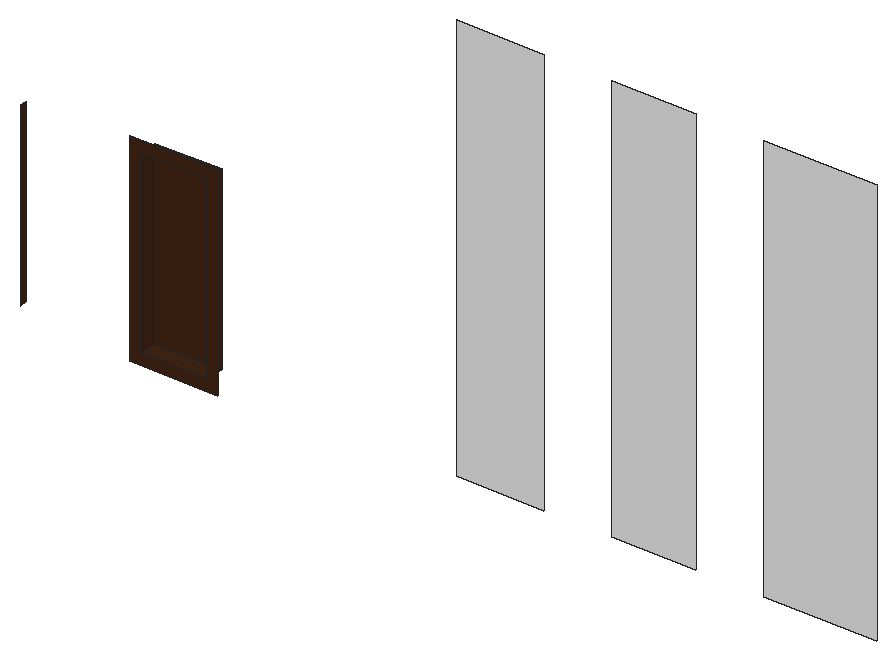
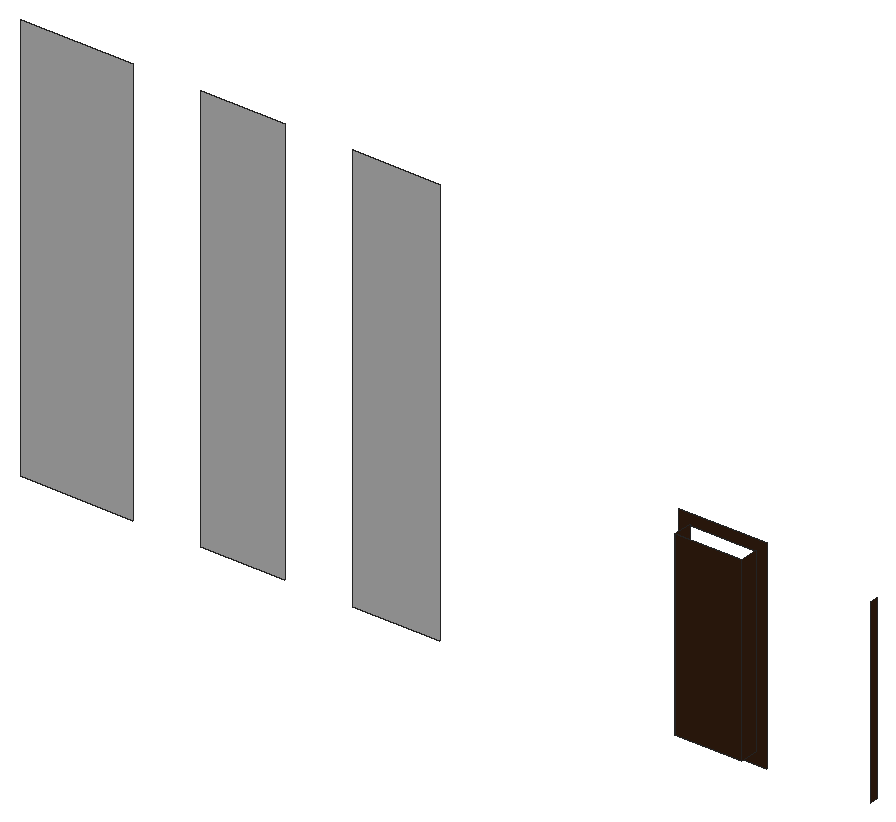
# SketchUp Ruby script. Lengths in inches.
U = 1.inch
M = Sketchup.active_model
def pt(a) = Geom::Point3d.new(a.map { |v| v * U })
def face(e, loops, mat)
  f = e.add_face(loops[0].map { |a| pt(a) })
  loops[1..].each { |l| e.add_face(l.map { |a| pt(a) }).erase! }
  f.material = f.back_material = mat if mat
  f
end
# faces: each face lists its corners as indices into pts; further lists are holes
def faces(e, pts, list, mat = nil) = list.each { |f| face(e, (f[0].is_a?(Array) ? f : [f]).map { |l| l.map { |i| pts[i] } }, mat) }
# xy, xz, yz: faces in a plane at the given z, y or x. An outline is a flat list of corners, or four numbers for a rectangle; further outlines are holes
def ring(l) = l.size == 4 ? [[l[0], l[1]], [l[2], l[1]], [l[2], l[3]], [l[0], l[3]]] : l.each_slice(2).to_a
def flat(e, list, mat, &to3) = list.each { |f| face(e, (f[0].is_a?(Array) ? f : [f]).map { |l| ring(l).map { |u, v| to3.(u, v) } }, mat) }
def xy(e, z, list, mat = nil) = flat(e, list, mat) { |x, y| [x, y, z] }
def xz(e, y, list, mat = nil) = flat(e, list, mat) { |x, z| [x, y, z] }
def yz(e, x, list, mat = nil) = flat(e, list, mat) { |y, z| [x, y, z] }
def lines(e, pts, list) = list.each { |a, b| e.add_line(pt(pts[a]), pt(pts[b])) }
# prism: a flat outline (further loops are holes) pulled along v
def prism(e, loops, v, mat = nil)
  f = face(e, loops, mat); d = Geom::Vector3d.new(v.map { |x| x * U })
  f.pushpull(f.normal.samedirection?(d) ? d.length : -d.length)
end
def box(e, o, s, mat = nil) = prism(e, [[o, [o[0] + s[0], o[1], o[2]], [o[0] + s[0], o[1] + s[1], o[2]], [o[0], o[1] + s[1], o[2]]]], [0, 0, s[2]], mat)
def at(x, y, z, deg = 0) = Geom::Transformation.translation(pt([x, y, z])) * Geom::Transformation.rotation(ORIGIN, Z_AXIS, deg.degrees)
def axes(o, x, y, z) = Geom::Transformation.new([*x, 0, *y, 0, *z, 0, *pt(o).to_a, 1])
def part(name) = M.definitions.add(name)
# library, detail: a bought-in or finely detailed component or shape, given as its bounding box
def library(name, o, s) = part(name).tap { |d| box(d.entities, o, s) }
def detail(e, o, s) = box(e.add_group.entities, o, s)
def put(e, d, t, mat = nil) = e.add_instance(d, t).tap { |i| i.material = mat if mat }
def group(e, t, mat = nil) = e.add_group.tap { |g| g.transformation = t; g.material = mat if mat }.entities
root = M.entities
M.materials.add("[Mirror 02]").color = [229, 229, 229]
M.materials.add("[Wood Veneer 01]").color = [66, 38, 20]
xy(root,135.37,[[292.21,244.48,321.41,252.61]],"[Wood Veneer 01]")
xz(root,244.48,[[[287.31,130.46,326.31,219.72],[292.21,135.37,321.41,214.82]]],"[Wood Veneer 01]")
xz(root,248.23,[[428.85,132.9375,467.73,313.62],[497.52,132.9375,534.68,313.62],[564.8,132.9375,614.56,313.62]],"[Mirror 02]")
xz(root,252.61,[[292.21,135.37,321.41,214.82]],"[Wood Veneer 01]")
yz(root,239.03,[[244.48,135.37,247.79,214.82]],"[Wood Veneer 01]")
yz(root,292.21,[[244.48,135.37,252.61,214.82]],"[Wood Veneer 01]")
yz(root,321.41,[[244.48,135.37,252.61,214.82]],"[Wood Veneer 01]")
